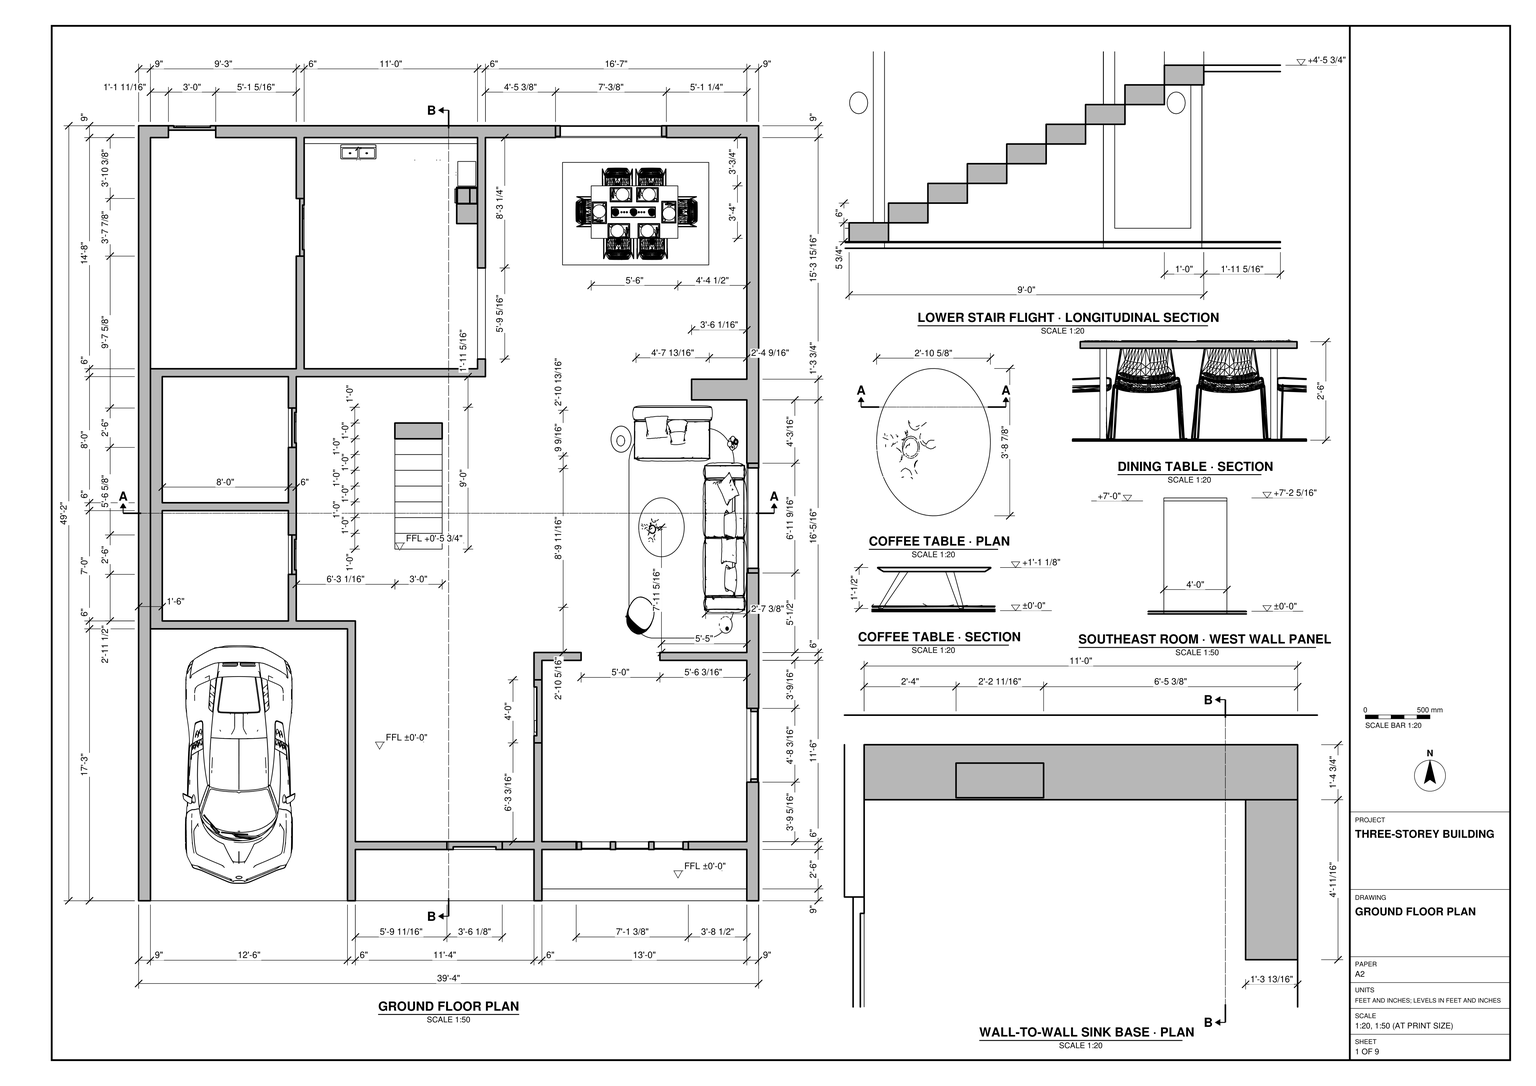
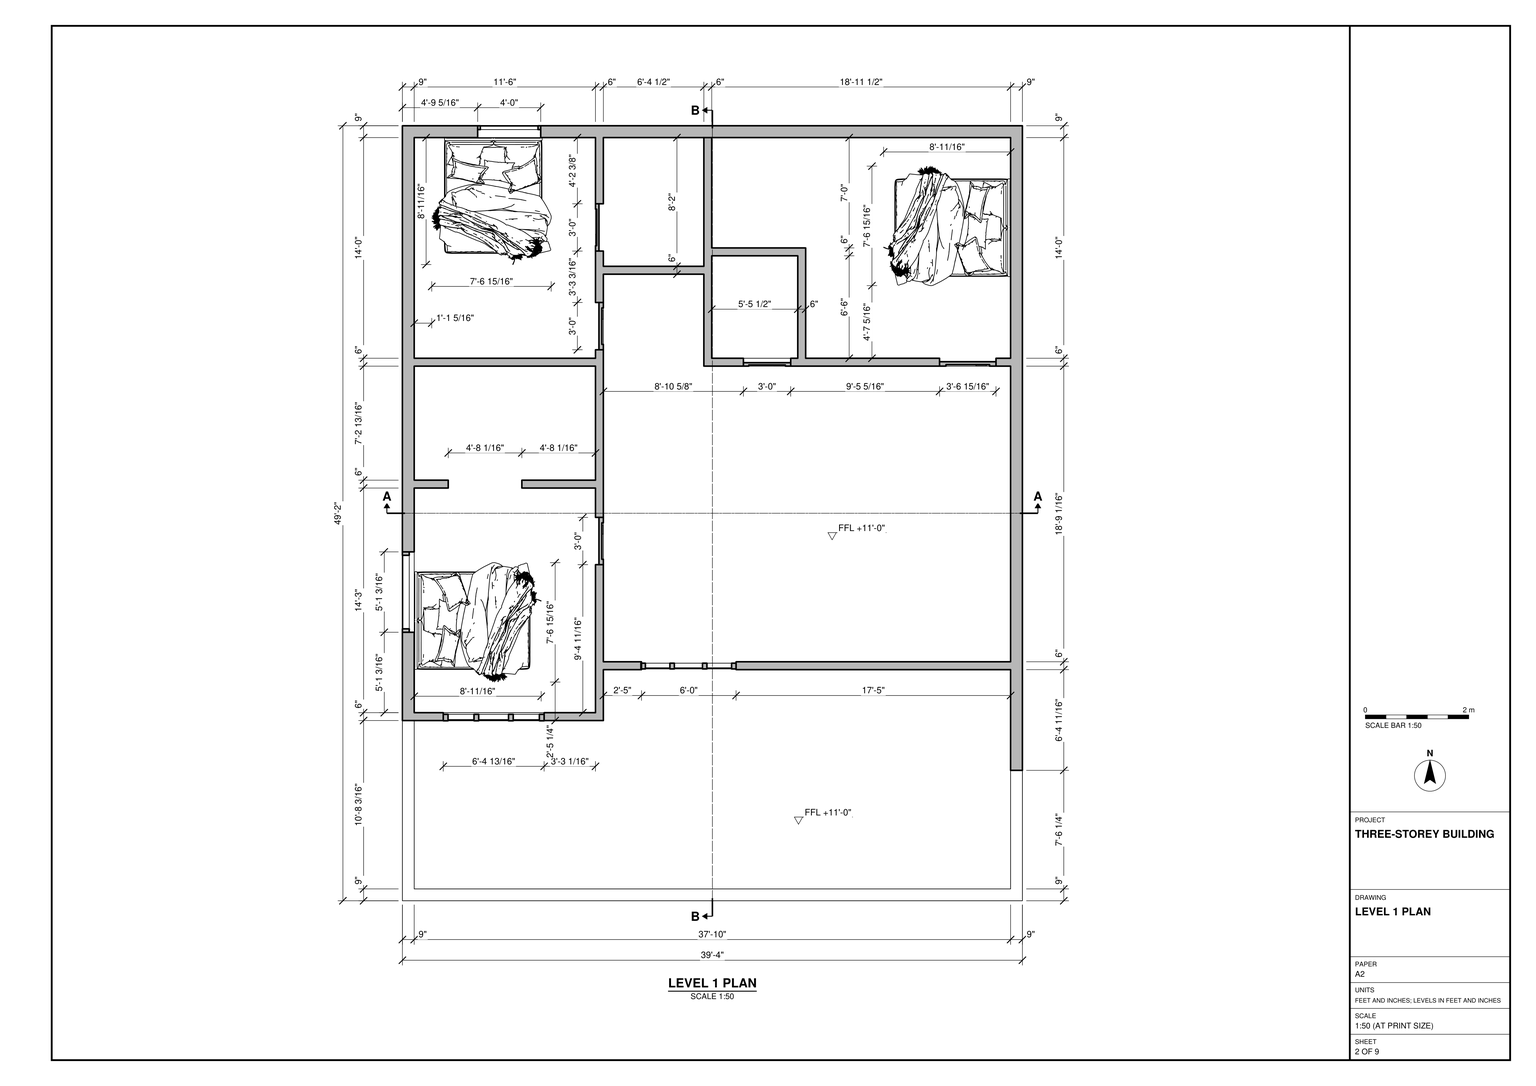
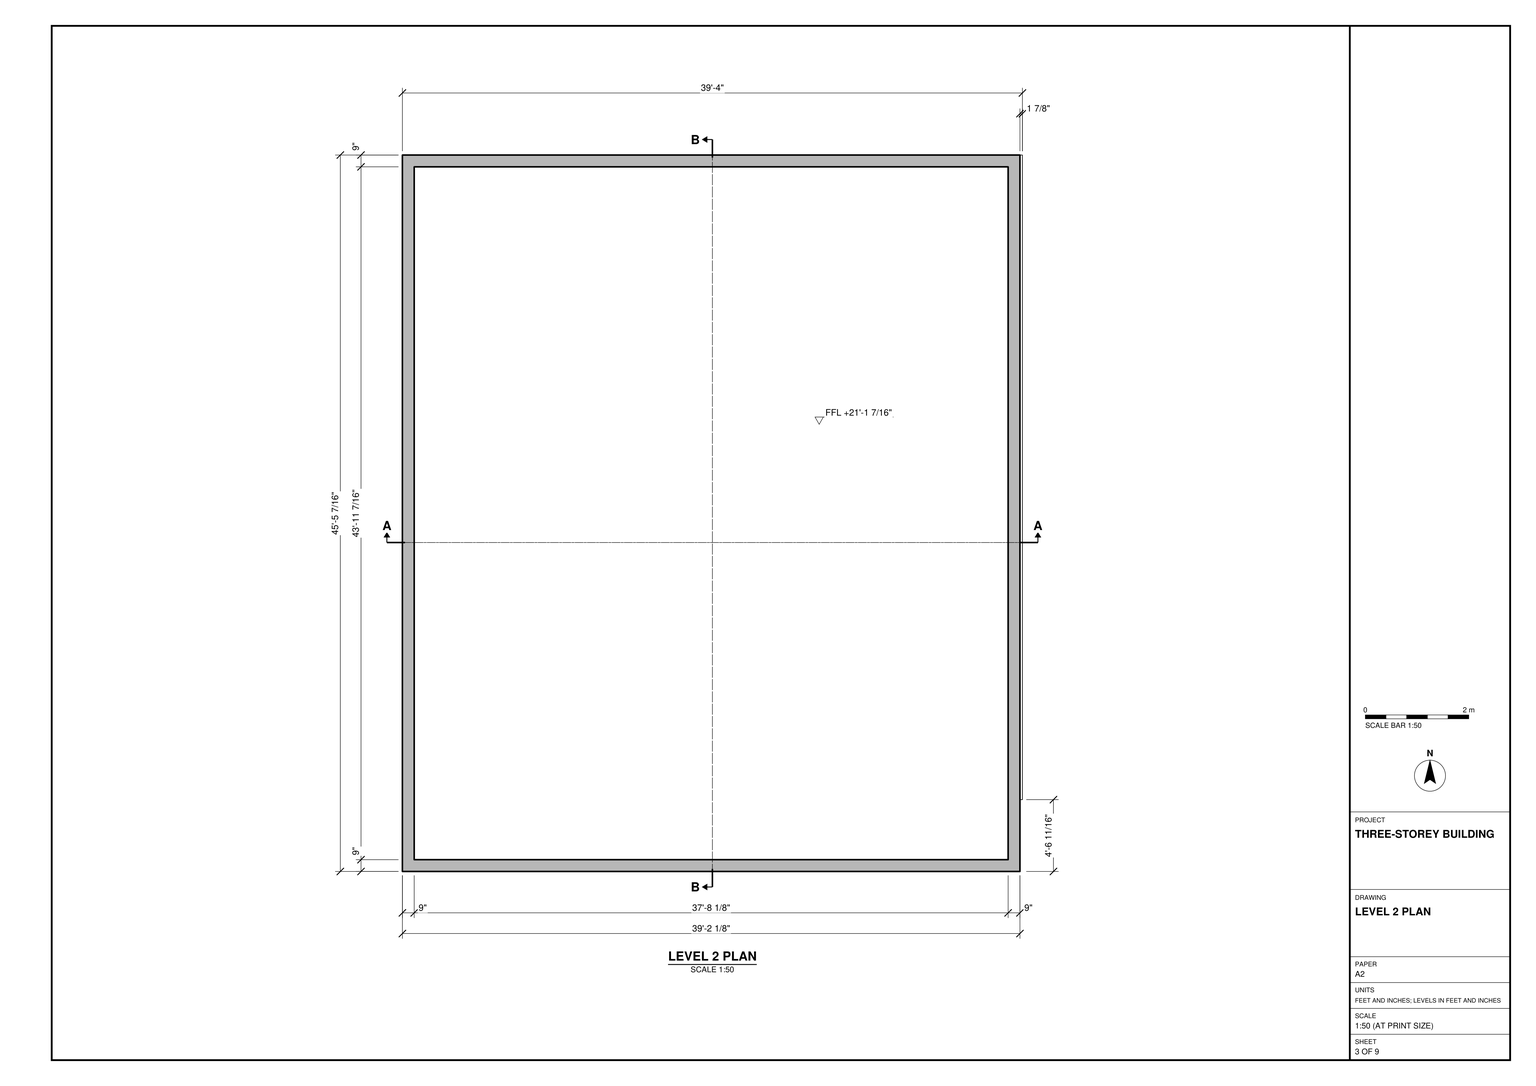
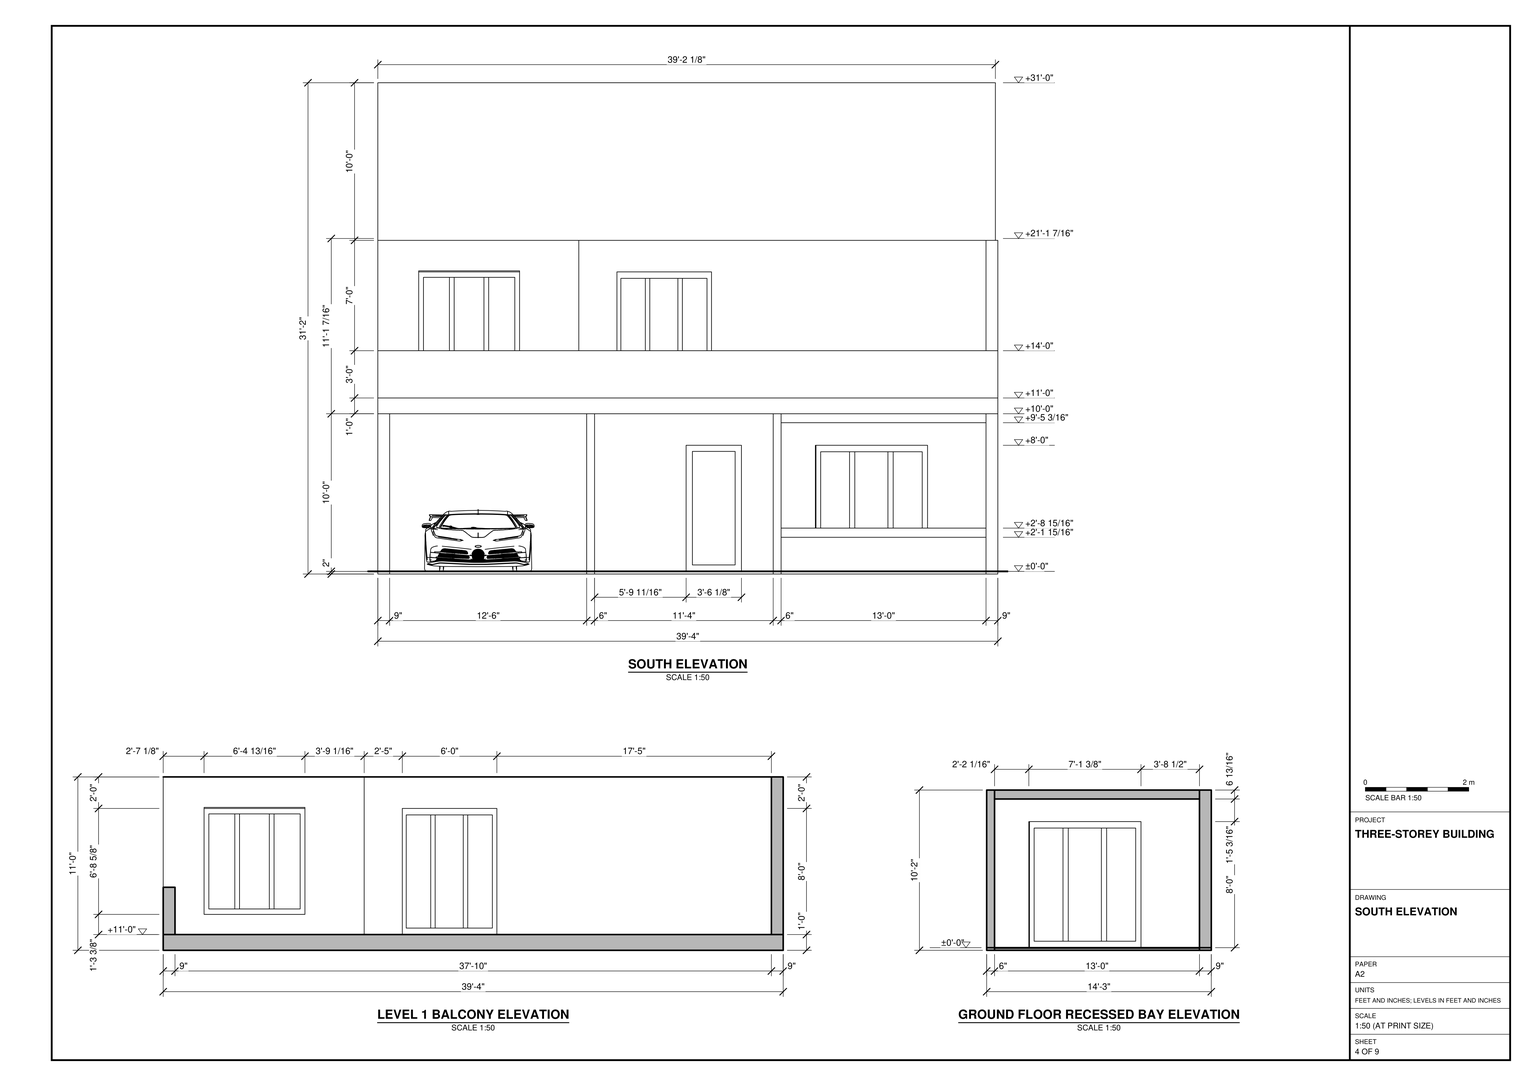
Build the three-storey residential building in SketchUp using task_files/diagram_01.pdf. Work in feet and inches. With north at the top of the plans, set out an overall east–west width of 39'-4" along X, a north–south depth of 49'-2" along Y and a total height of 31'-2". Use storey levels of ±0'-0", +10'-0" and +21'-1 7/16" relative to the ground floor.

Follow each floor plan for the wall positions and thicknesses, including the 9" perimeter walls and 6" partitions where indicated. Model the door and window openings, floor slabs, stairs, upper perimeter walls and roof edges as drawn. Preserve the stepped south edge of the enclosed rooms on the first upper floor rather than repeating the ground-floor layout.

On the ground floor, place the car in the southwest bay and the lower stair flight near the centre. Fit the kitchen with the wall-to-wall sink base and its return. Place the dining set in the northeast and arrange the sofas and coffee table farther south along the east side. Include the west wall panel in the southeast room. On the first upper floor, position and orient the beds to match the bedroom plan. Decor and loose items, including the car and appliances, may be any suitable library components.

Keep shell elements such as walls, slabs and roof separate as groups or components. Group each furniture or joinery piece separately and use components for repeated parts. Save one SketchUp model as output_files/three_storey_residential_building_and_its_furnishings.skp.

# SketchUp Ruby script. Lengths in inches.
U = 1.inch
M = Sketchup.active_model
def pt(a) = Geom::Point3d.new(a.map { |v| v * U })
def face(e, loops, mat)
  f = e.add_face(loops[0].map { |a| pt(a) })
  loops[1..].each { |l| e.add_face(l.map { |a| pt(a) }).erase! }
  f.material = f.back_material = mat if mat
  f
end
# faces: each face lists its corners as indices into pts; further lists are holes
def faces(e, pts, list, mat = nil) = list.each { |f| face(e, (f[0].is_a?(Array) ? f : [f]).map { |l| l.map { |i| pts[i] } }, mat) }
# xy, xz, yz: faces in a plane at the given z, y or x. An outline is a flat list of corners, or four numbers for a rectangle; further outlines are holes
def ring(l) = l.size == 4 ? [[l[0], l[1]], [l[2], l[1]], [l[2], l[3]], [l[0], l[3]]] : l.each_slice(2).to_a
def flat(e, list, mat, &to3) = list.each { |f| face(e, (f[0].is_a?(Array) ? f : [f]).map { |l| ring(l).map { |u, v| to3.(u, v) } }, mat) }
def xy(e, z, list, mat = nil) = flat(e, list, mat) { |x, y| [x, y, z] }
def xz(e, y, list, mat = nil) = flat(e, list, mat) { |x, z| [x, y, z] }
def yz(e, x, list, mat = nil) = flat(e, list, mat) { |y, z| [x, y, z] }
def lines(e, pts, list) = list.each { |a, b| e.add_line(pt(pts[a]), pt(pts[b])) }
# prism: a flat outline (further loops are holes) pulled along v
def prism(e, loops, v, mat = nil)
  f = face(e, loops, mat); d = Geom::Vector3d.new(v.map { |x| x * U })
  f.pushpull(f.normal.samedirection?(d) ? d.length : -d.length)
end
def box(e, o, s, mat = nil) = prism(e, [[o, [o[0] + s[0], o[1], o[2]], [o[0] + s[0], o[1] + s[1], o[2]], [o[0], o[1] + s[1], o[2]]]], [0, 0, s[2]], mat)
def at(x, y, z, deg = 0) = Geom::Transformation.translation(pt([x, y, z])) * Geom::Transformation.rotation(ORIGIN, Z_AXIS, deg.degrees)
def axes(o, x, y, z) = Geom::Transformation.new([*x, 0, *y, 0, *z, 0, *pt(o).to_a, 1])
def part(name) = M.definitions.add(name)
# library, detail: a bought-in or finely detailed component or shape, given as its bounding box
def library(name, o, s) = part(name).tap { |d| box(d.entities, o, s) }
def detail(e, o, s) = box(e.add_group.entities, o, s)
def put(e, d, t, mat = nil) = e.add_instance(d, t).tap { |i| i.material = mat if mat }
def group(e, t, mat = nil) = e.add_group.tap { |g| g.transformation = t; g.material = mat if mat }.entities
root = M.entities
M.materials.add("[Carrera Marble]").color = [207, 207, 207]
M.materials.add("[Color A01]").color = [255, 204, 204]
M.materials.add("[Color C08]").color = [102, 51, 0]
M.materials.add("[Color E01]").color = [255, 255, 204]
M.materials.add("[Color G01]").color = [204, 255, 204]
M.materials.add("[Color J01]").color = [229, 204, 255]
M.materials.add("[Color M08]").color = [30, 30, 30]
M.materials.add("[Concrete Pavers Block Multi]").color = [124, 140, 145]
M.materials.add("[Concrete Scored Jointless]").color = [140, 133, 127]
M.materials.add("[Formica Laminate Light]").color = [213, 189, 164]
M.materials.add("[Marble Carrara Gold Floor Tile]").color = [225, 223, 217]
M.materials.add("[Resin Blue]").color = [171, 210, 241]
M.materials.add("[Resin Turquoise]").color = [117, 218, 223]
M.materials.add("[Stone Coursed Rough]").color = [165, 160, 130]
M.materials.add("[Translucent Glass Blue]").color = [100, 149, 237]
M.materials.add("[Translucent Glass Gray]").color = [128, 128, 128]
M.materials.add("[Wood Floor]").color = [155, 105, 61]
c1 = library("L-shaped kitchen",[55.71,-118.11,21.3],[196.85,118.11,96.45])
c2 = library("28",[-28.6,-106.68,0],[90.94,96.67,40.97])
c3 = library("Sofa set Collection\#1",[635.72,692.31,0],[158.93,122.75,75.39])
c4 = library("skp3430",[-10.67,-22.6875,-0.04],[21.34,45.28,11.76])
c5 = library("Dining Set",[0,0,0],[111.37,78.0625,43.36])
c6 = part("Group\#7")
xy(c6.entities,0,[[0,0,36,6]])
xy(c6.entities,4.09,[[4.09,0,31.91,2.0625]],"[Color C08]")
xy(c6.entities,79.91,[[4.09,0,31.91,2.0625]],"[Color C08]")
xy(c6.entities,84,[[0,0,36,6]],"[Color C08]")
xz(c6.entities,0,[[[0,0,36,84],[4.09,4.09,31.91,79.91]]],"[Color C08]")
xz(c6.entities,0.25,[[26.54,38.97,27.4,39.08,28.2,39.41,28.88,39.9375,29.41,40.625,29.74,41.42,29.85,42.28,29.74,43.14,29.41,43.9375,28.88,44.625,28.2,45.15,27.4,45.48,26.54,45.59,25.68,45.48,24.89,45.15,24.2,44.625,23.67,43.9375,23.34,43.14,23.23,42.28,23.34,41.42,23.67,40.625,24.2,39.9375,24.89,39.41,25.68,39.08]],"[Color C08]")
xz(c6.entities,2.0625,[[[4.09,4.09,31.91,79.91],[26.54,38.97,25.68,39.08,24.89,39.41,24.2,39.9375,23.67,40.625,23.34,41.42,23.23,42.28,23.34,43.14,23.67,43.9375,24.2,44.625,24.89,45.15,25.68,45.48,26.54,45.59,27.4,45.48,28.2,45.15,28.88,44.625,29.41,43.9375,29.74,43.14,29.85,42.28,29.74,41.42,29.41,40.625,28.88,39.9375,28.2,39.41,27.4,39.08]]],"[Wood Floor]")
xz(c6.entities,6,[[0,0,36,84]])
yz(c6.entities,0,[[0,0,6,84]],"[Color C08]")
yz(c6.entities,4.09,[[0,4.09,2.0625,79.91]],"[Color C08]")
yz(c6.entities,31.91,[[0,4.09,2.0625,79.91]],"[Color C08]")
yz(c6.entities,36,[[0,0,6,84]],"[Color C08]")
p = [[25.68,2.0625,39.08],[26.54,2.0625,38.97],[26.54,0.25,38.97],[25.68,0.25,39.08],[27.4,2.0625,39.08],[27.4,0.25,39.08],
  [24.89,2.0625,39.41],[24.89,0.25,39.41],[28.2,2.0625,39.41],[28.2,0.25,39.41],[24.2,2.0625,39.9375],[24.2,0.25,39.9375],
  [28.88,2.0625,39.9375],[28.88,0.25,39.9375],[23.67,2.0625,40.625],[23.67,0.25,40.625],[29.41,2.0625,40.625],[29.41,0.25,40.625],
  [23.34,2.0625,41.42],[23.34,0.25,41.42],[29.74,2.0625,41.42],[29.74,0.25,41.42],[23.23,2.0625,42.28],[23.23,0.25,42.28],
  [29.85,2.0625,42.28],[29.85,0.25,42.28],[23.34,2.0625,43.14],[23.34,0.25,43.14],[29.74,2.0625,43.14],[29.74,0.25,43.14],
  [23.67,2.0625,43.9375],[23.67,0.25,43.9375],[29.41,2.0625,43.9375],[29.41,0.25,43.9375],[24.2,2.0625,44.625],[24.2,0.25,44.625],
  [28.88,2.0625,44.625],[28.88,0.25,44.625],[24.89,2.0625,45.15],[24.89,0.25,45.15],[28.2,2.0625,45.15],[28.2,0.25,45.15],
  [25.68,2.0625,45.48],[25.68,0.25,45.48],[27.4,2.0625,45.48],[27.4,0.25,45.48],[26.54,2.0625,45.59],[26.54,0.25,45.59]]
faces(c6.entities,p,[[0,1,2,3],[1,4,5,2],[6,0,3,7],[4,8,9,5],[10,6,7,11],[8,12,13,9],[14,10,11,15],[12,16,17,13],
  [18,14,15,19],[16,20,21,17],[22,18,19,23],[20,24,25,21],[26,22,23,27],[24,28,29,25],[30,26,27,31],[28,32,33,29],
  [34,30,31,35],[32,36,37,33],[38,34,35,39],[36,40,41,37],[42,38,39,43],[40,44,45,41],[46,42,43,47],[44,46,47,45]],"[Color C08]")
c7 = part("Group\#8")
box(c7.entities,[0,0,0],[36,12,6])
c8 = part("Group\#10")
put(c8.entities,c7,at(0,24,12))
put(c8.entities,c7,at(0,96,48))
put(c8.entities,c7,at(0,36,18))
put(c8.entities,c7,at(0,48,24))
put(c8.entities,c7,at(0,72,36))
put(c8.entities,c7,at(0,84,42))
put(c8.entities,c7,at(0,0,0))
put(c8.entities,c7,at(0,12,6))
put(c8.entities,c7,at(0,60,30))
c9 = part("Group\#14")
xy(c9.entities,0,[[0,0,8.11,83.5625]])
xy(c9.entities,3.3125,[[7.9,3.57,8.11,80]])
xy(c9.entities,3.3125,[[0,3.57,7.9,80]],"[Color C08]")
xy(c9.entities,44.6875,[[0,3.57,7.9,80],[7.9,3.57,8.11,80]])
xy(c9.entities,48,[[0,0,8.11,83.5625]],"[Color C08]")
xz(c9.entities,0,[[0,0,8.11,48]],"[Color C08]")
xz(c9.entities,3.57,[[7.9,3.3125,8.11,44.6875]])
xz(c9.entities,3.57,[[0,3.3125,7.9,44.6875]],"[Color C08]")
xz(c9.entities,80,[[7.9,3.3125,8.11,44.6875]])
xz(c9.entities,80,[[0,3.3125,7.9,44.6875]],"[Color C08]")
xz(c9.entities,83.5625,[[0,0,8.11,48]],"[Color C08]")
yz(c9.entities,0,[[[0,0,83.5625,48],[3.57,3.3125,80,44.6875]]],"[Color C08]")
yz(c9.entities,7.9,[[3.57,3.3125,80,44.6875]],"[Translucent Glass Gray]")
yz(c9.entities,8.11,[[[0,0,83.5625,48],[3.57,3.3125,80,44.6875]]],"[Color C08]")
c10 = library("Group\#11",[0,0,0],[343,572,6.8125])
c11 = part("Group\#12")
xy(c11.entities,0,[[0,0,77.625,5.875]])
xy(c11.entities,3.68,[[3.68,0,23.65,0.75],[23.65,0,27.29,5.875],[27.29,0,50.21,0.75],[50.21,0,53.85,5.875],[53.85,0,73.95,0.75],
  [3.68,0.75,23.65,5.875],[27.29,0.75,50.21,5.875],[53.85,0.75,73.95,5.875]],"[Color C08]")
xy(c11.entities,68.14,[[3.68,0,23.65,0.75],[23.65,0,27.29,5.875],[27.29,0,50.21,0.75],[50.21,0,53.85,5.875],[53.85,0,73.95,0.75],
  [3.68,0.75,23.65,5.875],[27.29,0.75,50.21,5.875],[53.85,0.75,73.95,5.875]])
xy(c11.entities,71.8125,[[0,0,77.625,5.875]],"[Color C08]")
xz(c11.entities,0,[[[0,0,77.625,71.8125],[3.68,3.68,73.95,68.14]],[23.65,3.68,27.29,68.14],[50.21,3.68,53.85,68.14]],"[Color C08]")
xz(c11.entities,0.75,[[3.68,3.68,23.65,68.14],[27.29,3.68,50.21,68.14],[53.85,3.68,73.95,68.14]],"[Translucent Glass Gray]")
xz(c11.entities,5.875,[[[0,0,77.625,71.8125],[3.68,3.68,73.95,68.14]],[23.65,3.68,27.29,68.14],[50.21,3.68,53.85,68.14]],"[Color C08]")
yz(c11.entities,0,[[0,0,5.875,71.8125]],"[Color C08]")
yz(c11.entities,3.68,[[0,3.68,0.75,68.14],[0.75,3.68,5.875,68.14]],"[Color C08]")
yz(c11.entities,23.65,[[0,3.68,0.75,68.14]])
yz(c11.entities,23.65,[[0.75,3.68,5.875,68.14]],"[Color C08]")
yz(c11.entities,27.29,[[0,3.68,0.75,68.14],[0.75,3.68,5.875,68.14]],"[Color C08]")
yz(c11.entities,50.21,[[0,3.68,0.75,68.14],[0.75,3.68,5.875,68.14]],"[Color C08]")
yz(c11.entities,53.85,[[0,3.68,0.75,68.14],[0.75,3.68,5.875,68.14]],"[Color C08]")
yz(c11.entities,73.95,[[0,3.68,0.75,68.14],[0.75,3.68,5.875,68.14]],"[Color C08]")
yz(c11.entities,77.625,[[0,0,5.875,71.8125]],"[Color C08]")
c12 = part("Group\#4")
xy(c12.entities,0,[[0,0,8.11,83.5625]])
xy(c12.entities,3.3125,[[7.9,3.57,8.11,80]])
xy(c12.entities,3.3125,[[0,3.57,7.9,80]],"[Color C08]")
xy(c12.entities,44.6875,[[0,3.57,7.9,80],[7.9,3.57,8.11,80]])
xy(c12.entities,48,[[0,0,8.11,83.5625]],"[Color C08]")
xz(c12.entities,0,[[0,0,8.11,48]],"[Color C08]")
xz(c12.entities,3.57,[[7.9,3.3125,8.11,44.6875]])
xz(c12.entities,3.57,[[0,3.3125,7.9,44.6875]],"[Color C08]")
xz(c12.entities,80,[[7.9,3.3125,8.11,44.6875]])
xz(c12.entities,80,[[0,3.3125,7.9,44.6875]],"[Color C08]")
xz(c12.entities,83.5625,[[0,0,8.11,48]],"[Color C08]")
yz(c12.entities,0,[[[0,0,83.5625,48],[3.57,3.3125,80,44.6875]]],"[Color C08]")
yz(c12.entities,7.9,[[3.57,3.3125,80,44.6875]],"[Translucent Glass Gray]")
yz(c12.entities,8.11,[[[0,0,83.5625,48],[3.57,3.3125,80,44.6875]]],"[Color C08]")
xy(root,252,[[0,44.5625,470.125,590]])
xy(root,253.4375,[[9,53.5625,461.125,581]])
xy(root,372,[[[0,44.5625,470.125,590],[9,53.5625,461.125,581]]])
xz(root,44.5625,[[0,252,470.125,372]],"[Color G01]")
xz(root,53.5625,[[9,253.4375,461.125,372]])
xz(root,581,[[9,253.4375,461.125,372]])
xz(root,590,[[0,252,470.125,372]])
yz(root,0,[[44.5625,252,590,372]],"[Color G01]")
yz(root,9,[[53.5625,253.4375,581,372]])
yz(root,461.125,[[53.5625,253.4375,581,372]])
yz(root,470.125,[[44.5625,252,590,372]],"[Color G01]")
# 1 loose lines left out
put(root,c1,axes([88.64,576.42,-21.03],[0.67056,0,0],[0,0.51559,0],[0,0,0.98757]))
put(root,c2,at(50.9375,591.01,132))
put(root,c3,axes([-237.95,1084.5,0],[0,-1.1131,0],[0.86,0,0],[0,0,1]))
put(root,c4,axes([76.36,103.91,0.17],[4,0,0],[0,4,0],[0,0,4]))
put(root,c5,at(322.6875,484.04,0))
put(root,c2,at(-1.01,195.0625,132,90))
put(root,c2,at(473.01,530.66,132,-90))
g1 = group(root,at(234.6875,39,0.24))
xy(g1,0,[[0,0,42.125,6]])
xy(g1,4.66,[[4.79,0,37.34,2.0625]],"[Color C08]")
xy(g1,91.1,[[4.79,0,37.34,2.0625]],"[Color C08]")
xy(g1,95.76,[[0,0,42.125,6]],"[Color C08]")
xz(g1,0,[[[0,0,42.125,95.76],[4.79,4.66,37.34,91.1]]],"[Color C08]")
xz(g1,2.0625,[[4.79,4.66,37.34,91.1]],"[Translucent Glass Blue]")
xz(g1,6,[[0,0,42.125,95.76]],"[Translucent Glass Blue]")
yz(g1,0,[[0,0,6,95.76]],"[Color C08]")
yz(g1,4.79,[[0,4.66,2.0625,91.1]],"[Color C08]")
yz(g1,37.34,[[0,4.66,2.0625,91.1]],"[Color C08]")
yz(g1,42.125,[[0,0,6,95.76]],"[Color C08]")
put(root,c6,axes([301,168.1875,0],[0,-1.33333,0],[1,0,0],[0,0,1.02728]))
put(root,c6,axes([126,490.74,0],[0,1.21875,0],[-0.56,0,0],[0,0,1]))
put(root,c6,axes([58.6875,590,0],[-1,0,0],[0,-0.56,0],[0,0,1]))
g2 = group(root,at(156.39,267.6875,-0.25))
box(g2,[0,108,52.0625],[74.6875,23.3125,1.9375])
put(g2,c8,at(38.6875,0,0))
put(g2,c8,at(36.4375,108,54,-180))
g3 = group(root,at(333.09,39,0))
xy(g3,0,[[0,0,85.39,5.875]])
xy(g3,4.92,[[4.05,0,26.02,0.75],[26.02,0,30.01,5.875],[30.01,0,55.24,0.75],[55.24,0,59.23,5.875],[59.23,0,81.34,0.75],
  [4.05,0.75,26.02,5.875],[30.01,0.75,55.24,5.875],[59.23,0.75,81.34,5.875]],"[Color C08]")
xy(g3,91.08,[[4.05,0,26.02,0.75],[26.02,0,30.01,5.875],[30.01,0,55.24,0.75],[55.24,0,59.23,5.875],[59.23,0,81.34,0.75],
  [4.05,0.75,26.02,5.875],[30.01,0.75,55.24,5.875],[59.23,0.75,81.34,5.875]])
xy(g3,96,[[0,0,85.39,5.875]],"[Color C08]")
xz(g3,0,[[[0,0,85.39,96],[4.05,4.92,81.34,91.08]],[26.02,4.92,30.01,91.08],[55.24,4.92,59.23,91.08]],"[Color C08]")
xz(g3,0.75,[[4.05,4.92,26.02,91.08],[30.01,4.92,55.24,91.08],[59.23,4.92,81.34,91.08]],"[Translucent Glass Gray]")
xz(g3,5.875,[[[0,0,85.39,96],[4.05,4.92,81.34,91.08]],[26.02,4.92,30.01,91.08],[55.24,4.92,59.23,91.08]],"[Color C08]")
yz(g3,0,[[0,0,5.875,96]],"[Color C08]")
yz(g3,4.05,[[0,4.92,0.75,91.08],[0.75,4.92,5.875,91.08]],"[Color C08]")
yz(g3,26.02,[[0,4.92,0.75,91.08]])
yz(g3,26.02,[[0.75,4.92,5.875,91.08]],"[Color C08]")
yz(g3,30.01,[[0,4.92,0.75,91.08],[0.75,4.92,5.875,91.08]],"[Color C08]")
yz(g3,55.24,[[0,4.92,0.75,91.08],[0.75,4.92,5.875,91.08]],"[Color C08]")
yz(g3,59.23,[[0,4.92,0.75,91.08],[0.75,4.92,5.875,91.08]],"[Color C08]")
yz(g3,81.34,[[0,4.92,0.75,91.08],[0.75,4.92,5.875,91.08]],"[Color C08]")
yz(g3,85.39,[[0,0,5.875,96]],"[Color C08]")
put(root,c9,axes([466.08,90.29,36],[0.6424,0,0],[0,0.6722,0],[0,0,1]))
put(root,c9,axes([401.74,581.89,36],[0,1,0],[-1.01,0,0],[0,0,1]))
put(root,c9,at(463.89,249.52,35.62))
put(root,c6,axes([120,248.47,0],[0,0.83333,0],[-0.56,0,0],[0,0,1]))
put(root,c6,axes([120,345.16,0],[0,0.83333,0],[-0.56,0,0],[0,0,1]))
put(root,c10,at(120,9.4375,113.1875))
put(root,c11,axes([31.12,136.99,147.35],[0.98929,0,0],[0,0.84,0],[0,0,1.12292]))
put(root,c9,axes([5.21,265.6,168],[-0.6424,0,0],[0,-0.73246,0],[0,0,1]))
put(root,c12,axes([105.31,587.08,168],[0,0.36,0],[-0.57442,0,0],[0,0,0.9864]))
put(root,c12,axes([200.85,588.1,201.9375],[0,0.234,0],[-0.28721,0,0],[0,0,0.51724]))
put(root,c6,axes([153,255.87,132],[0,1,0],[-0.56,0,0],[0,0,1]))
put(root,c6,axes([153,419.45,132],[0,1,0],[-0.56,0,0],[0,0,1]))
put(root,c6,axes([408.93,407,132],[1.19343,0,0],[0,0.56,0],[0,0,1]))
put(root,c6,axes([259.62,407,132],[1,0,0],[0,0.43999,0],[0,0,1]))
put(root,c6,axes([147,530.61,132],[0,-1,0],[0.43999,0,0],[0,0,1]))
put(root,c11,axes([181.58,176.48,132],[0.9333,0,0],[0,0.7476,0],[0,0,1.33681]))
g4 = group(root,at(0,0,-2),"[Color G01]")
xy(g4,0,[[0,0,0,590,9.3125,590,9.3125,581,9,581,9,0],[159,0,159,207,9.3125,207,9.3125,405,120,405,120,490.74,126,490.74,126,405,258,405,258,412.4,264,412.4,264,399,120,399,120,375.1,114,375.1,114,399,18,399,18,303,114,303,114,345.1,120,345.1,120,278.47,114,278.47,114,297,18,297,18,213,114,213,114,248.47,120,248.47,120,213,165,213,165,45,234.6875,45,234.6875,39,165,39,165,0],[301,0,301,39,276.8125,39,276.8125,45,301,45,301,120.1875,307,120.1875,307,45,333.57,45,333.57,39,307,39,307,0],[307,0,463,9],[463,0,463,39,418.48,39,418.48,45,463,45,463,90.29,472,90.29,472,0],
  [[307,9,307,39,333.57,39,333.57,45,307,45,307,120.1875,301,120.1875,301,45,165,45,165,213,120,213,120,399,264,399,264,581,317.34,581,317.34,590,401.89,590,401.89,581,463,581,463,397.04,420.9375,397.04,420.9375,381.29,463,381.29,463,189,396.83,189,396.83,183,463,183,463,146.46,472,146.46,472,90.29,463,90.29,463,45,418.48,45,418.48,39,463,39,463,9],[301,168.1875,307,168.1875,307,183,336.83,183,336.83,189,301,189]],[234.6875,39,276.8125,45],[463,146.46,463,183,396.83,183,396.83,189,463,189,463,333.08,472,333.08,472,146.46],[301,168.1875,301,189,336.83,189,336.83,183,307,183,307,168.1875],[114,248.47,120,278.47],
  [463,333.08,463,381.29,420.9375,381.29,420.9375,397.04,463,397.04,463,581,401.89,581,401.89,590,472,590,472,333.08],[114,345.1,120,375.1],[258,412.4,264,481.74],[258,481.74,258,581,126,581,126,534.62,120,534.62,120,581,58.6875,581,58.6875,590,317.34,590,317.34,581,264,581,264,481.74],[9.3125,581,22.6875,590]])
xy(g4,0,[[9,0,159,207]],"[Concrete Scored Jointless]")
xy(g4,0,[[165,0,301,39],[18,213,114,297],[18,303,114,399],[9.3125,405,9.3125,581,22.6875,581,22.6875,590,58.6875,590,58.6875,581,120,581,120,534.62,126,534.62,126,581,258,581,258,405,126,405,126,490.74,120,490.74,120,405]],"[Marble Carrara Gold Floor Tile]")
xy(g4,1.75,[[[307,9,463,9,463,39,418.48,39,418.48,45,463,45,463,90.29,472,90.29,472,146.46,463,146.46,463,183,396.83,183,396.83,189,463,189,463,381.29,420.9375,381.29,420.9375,397.04,463,397.04,463,581,401.89,581,401.89,590,317.34,590,317.34,581,264,581,264,399,120,399,120,213,165,213,165,45,301,45,301,120.1875,307,120.1875,307,45,333.57,45,333.57,39,307,39],[301,168.1875,301,189,336.83,189,336.83,183,307,183,307,168.1875]]])
xy(g4,2,[[0,0,9,0,9,581,9.3125,581,9.3125,590,0,590],[159,0,165,0,165,39,234.6875,39,234.6875,45,165,45,165,213,120,213,120,248.47,114,248.47,114,213,18,213,18,297,114,297,114,278.47,120,278.47,120,345.1,114,345.1,114,303,18,303,18,399,114,399,114,375.1,120,375.1,120,399,264,399,264,412.4,258,412.4,258,405,126,405,126,490.74,120,490.74,120,405,9.3125,405,9.3125,207,159,207],[301,0,307,0,307,39,333.57,39,333.57,45,307,45,307,120.1875,301,120.1875,301,45,276.8125,45,276.8125,39,301,39],[463,0,472,0,472,90.29,463,90.29,463,45,418.48,45,418.48,39,463,39],[234.6875,39,276.8125,45],
  [463,90.29,472,146.46],[463,146.46,472,146.46,472,333.08,463,333.08,463,189,396.83,189,396.83,183,463,183],[301,168.1875,307,168.1875,307,183,336.83,183,336.83,189,301,189],[9,207,9.3125,405],[114,248.47,120,278.47],
  [463,333.08,472,333.08,472,590,401.89,590,401.89,581,463,581,463,397.04,420.9375,397.04,420.9375,381.29,463,381.29],[114,345.1,120,375.1],[258,481.74,264,481.74,264,581,317.34,581,317.34,590,58.6875,590,58.6875,581,120,581,120,534.62,126,534.62,126,581,258,581],[9.3125,581,22.6875,590],[317.34,581,401.89,590]])
xy(g4,2,[[18,213,114,297],[18,303,114,399]],"[Carrera Marble]")
xy(g4,2,[[165,0,301,39]],"[Color G01]")
xy(g4,2,[[9,0,9.3125,207],[9.3125,0,159,207]],"[Concrete Scored Jointless]")
xy(g4,2,[[9.3125,405,120,405,120,490.74,126,490.74,126,405,258,405,258,581,126,581,126,534.62,120,534.62,120,581,58.6875,581,58.6875,590,22.6875,590,22.6875,581,9.3125,581],[258,412.4,264,481.74]],"[Formica Laminate Light]")
xy(g4,2,[[[307,9,463,9,463,39,418.48,39,418.48,45,463,45,463,183,396.83,183,396.83,189,463,189,463,381.29,420.9375,381.29,420.9375,397.04,463,397.04,463,581,264,581,264,399,120,399,120,213,165,213,165,45,301,45,301,120.1875,307,120.1875,307,45,333.57,45,333.57,39,307,39],[301,168.1875,301,189,336.83,189,336.83,183,307,183,307,168.1875]],[9,405,9.3125,581]],"[Marble Carrara Gold Floor Tile]")
xy(g4,27.9375,[[307,0,463,9]])
xy(g4,34.9375,[[307,0,463,9]],"[Color G01]")
xy(g4,38,[[463,90.29,472,146.46],[463,249.52,472,333.08],[317.34,581,401.89,590]])
xy(g4,86,[[463,90.29,472,146.46],[336.83,183,396.83,189],[114,248.47,120,278.47],[463,249.52,472,333.08],[114,345.1,120,375.1],
  [120,490.74,126,534.62],[22.6875,581,58.6875,590],[317.34,581,401.89,590]])
xy(g4,98,[[234.6875,39,276.8125,45],[333.57,39,418.48,45]])
xy(g4,122,[[9,0,159,207],[165,0,301,39],[307,0,463,39],[165,45,301,45,301,189,463,189,463,381.29,420.9375,381.29,420.9375,397.04,463,397.04,463,581,264,581,264,481.74,258,481.74,258,581,126,581,126,405,258,405,258,412.4,264,412.4,264,399,120,399,120,213,165,213],[18,213,114,297],
  [18,303,114,399],[9,405,120,581]])
xy(g4,122,[[[0,0,9,0,9,581,120,581,120,405,9,405,9,207,159,207,159,0,165,0,165,39,301,39,301,0,307,0,307,39,463,39,463,0,472,0,472,590,0,590],[165,45,165,213,120,213,120,399,264,399,264,412.4,258,412.4,258,405,126,405,126,581,258,581,258,481.74,264,481.74,264,581,463,581,463,397.04,420.9375,397.04,420.9375,381.29,463,381.29,463,189,301,189,301,45],[307,45,463,183],[18,303,114,399],[18,213,114,297]]],"[Color G01]")
xy(g4,134,[[0,0,0,137.1875,9,137.1875,9,9,463,9,463,99.27,472,99.27,472,0],[463,99.27,463,175.9375,254.03,175.9375,254.03,181.9375,463,181.9375,463,407,451.9,407,451.9,413,463,413,463,581,200.85,581,200.85,590,472,590,472,99.27],[0,137.1875,0,265.6,9,265.6,9,143.1875,107.91,143.1875,107.91,137.1875],[107.91,137.1875,107.91,143.1875,147,143.1875,147,255.87,153,255.87,153,181.9375,182.03,181.9375,182.03,175.9375,153,175.9375,153,137.1875],[0,265.6,0,590,105.31,590,105.31,581,9,581,9,413,147,413,147,419.45,153,419.45,153,291.87,147,291.87,147,314.1875,90.95,314.1875,90.95,320.1875,147,320.1875,147,407,9,407,9,320.1875,34.9,320.1875,34.9,314.1875,9,314.1875,9,265.6],
  [229.5,407,229.5,477,153,477,153,455.45,147,455.45,147,494.61,153,494.61,153,483,229.5,483,229.5,581,235.5,581,235.5,497,307,497,307,413,408.93,413,408.93,407,295.62,407,295.62,413,301,413,301,491,235.5,491,235.5,413,259.62,413,259.62,407],[235.5,413,301,491],[147,530.61,147,581,105.31,581,105.31,590,200.85,590,200.85,581,153,581,153,530.61]])
xy(g4,134,[[9,9,463,9,463,175.9375,254.03,175.9375,254.03,181.9375,463,181.9375,463,407,451.9,407,451.9,413,463,413,463,581,235.5,581,235.5,497,307,497,307,413,408.93,413,408.93,407,295.62,407,295.62,413,259.62,413,259.62,407,229.5,407,229.5,477,153,477,153,455.45,147,455.45,147,494.61,153,494.61,153,483,229.5,483,229.5,581,153,581,153,530.61,147,530.61,147,581,9,581,9,413,147,413,147,419.45,153,419.45,153,291.87,147,291.87,147,314.1875,90.95,314.1875,90.95,320.1875,147,320.1875,147,407,9,407,9,320.1875,34.9,320.1875,34.9,314.1875,9,314.1875,9,143.1875,147,143.1875,147,255.87,153,255.87,153,181.9375,182.03,181.9375,182.03,175.9375,153,175.9375,153,137.1875,9,137.1875]],"[Marble Carrara Gold Floor Tile]")
xy(g4,149.35,[[31.12,137.1875,107.91,143.1875]])
xy(g4,170,[[0,204.39,9,265.6],[57.31,581,105.31,590]])
xy(g4,170,[[0,0,472,0,472,99.27,463,99.27,463,9,9,9,9,137.1875,0,137.1875]],"[Color M08]")
xy(g4,203.9375,[[176.85,581,200.85,590]])
xy(g4,218,[[0,204.39,9,265.6],[147,255.87,153,291.87],[34.9,314.1875,90.95,320.1875],[259.62,407,295.62,413],[408.93,407,451.9,413],
  [147,419.45,153,455.45],[147,494.61,153,530.61],[57.31,581,105.31,590]])
xy(g4,228.76,[[176.85,581,200.85,590]])
xy(g4,230,[[182.03,175.9375,254.03,181.9375]])
xy(g4,230.8125,[[31.12,137.1875,107.91,143.1875]])
xy(g4,254,[[[463,99.27,472,99.27,472,590,0,590,0,137.1875,153,137.1875,153,175.9375,463,175.9375],[153,181.9375,153,477,229.5,477,229.5,407,463,407,463,181.9375],[307,413,307,497,235.5,497,235.5,581,229.5,581,229.5,483,153,483,153,581,463,581,463,413],[9,143.1875,147,314.1875],[9,413,147,581],[9,320.1875,147,407],[235.5,413,301,491]]],"[Color E01]")
xz(g4,0,[[0,0,9,2],[301,0,307,2]])
xz(g4,0,[[9,0,159,2],[159,0,165,2],[165,0,301,2],[307,0,463,2],[463,0,472,2],
  [0,2,9,122],[159,2,165,122],[301,2,307,122],[463,2,472,122],[307,27.9375,463,34.9375],
  [0,122,472,134]],"[Color G01]")
xz(g4,0,[[307,2,463,27.9375]],"[Stone Coursed Rough]")
xz(g4,0,[[0,134,472,170]],"[Translucent Glass Blue]")
xz(g4,9,[[307,0,463,1.75],[307,1.75,463,2],[307,2,463,27.9375],[307,27.9375,463,34.9375]])
xz(g4,9,[[9,134,463,170]],"[Translucent Glass Blue]")
xz(g4,39,[[307,0,333.57,1.75],[418.48,0,463,1.75],[307,1.75,333.57,2],[418.48,1.75,463,2]])
xz(g4,39,[[165,2,234.6875,2,234.6875,98,276.8125,98,276.8125,2,301,2,301,122,165,122],[307,2,333.57,2,333.57,98,418.48,98,418.48,2,463,2,463,122,307,122]],"[Color G01]")
xz(g4,39,[[165,0,234.6875,2],[234.6875,0,276.8125,2],[276.8125,0,301,2]],"[Marble Carrara Gold Floor Tile]")
xz(g4,45,[[165,0,185.25,1.75],[185.25,0,234.6875,1.75],[234.6875,0,271.8125,1.75],[271.8125,0,276.8125,1.75],[276.8125,0,301,1.75],
  [307,0,333.57,1.75],[418.48,0,463,1.75],[165,1.75,185.25,2],[185.25,1.75,234.6875,2],[234.6875,1.75,271.8125,2],
  [271.8125,1.75,276.8125,2],[276.8125,1.75,301,2],[307,1.75,333.57,2],[418.48,1.75,463,2],[165,2,165,122,301,122,301,2,276.8125,2,276.8125,98,234.6875,98,234.6875,2]])
xz(g4,45,[[307,2,307,122,463,122,463,2,418.48,2,418.48,98,333.57,98,333.57,2]],"[Color J01]")
xz(g4,90.29,[[463,0,472,1.75],[463,1.75,472,2],[463,38,472,86]])
xz(g4,99.27,[[463,134,472,170]])
xz(g4,99.27,[[463,170,472,254]],"[Color G01]")
xz(g4,120.1875,[[301,0,307,1.75],[301,1.75,307,2],[301,2,301,88.29,307,86,307,2]])
xz(g4,137.1875,[[0,134,9,170]])
xz(g4,137.1875,[[[9,134,153,134,153,254,0,254,0,170,9,170],[31.12,149.35,107.91,230.8125]]],"[Color G01]")
xz(g4,143.1875,[[[9,134,147,254],[31.12,149.35,107.91,230.8125]]],"[Resin Turquoise]")
xz(g4,146.46,[[463,0,472,1.75],[463,1.75,472,2],[463,38,472,86]])
xz(g4,168.1875,[[301,0,307,1.75],[301,1.75,307,2],[301,2,301,88.29,307,86,307,2]])
xz(g4,175.9375,[[153,134,182.03,134,182.03,230,254.03,230,254.03,134,463,134,463,254,153,254]],"[Color G01]")
xz(g4,181.9375,[[153,134,153,254,463,254,463,134,254.03,134,254.03,230,182.03,230,182.03,134]],"[Color E01]")
xz(g4,183,[[307,0,336.83,1.75],[396.83,0,463,1.75],[307,1.75,336.83,2],[396.83,1.75,463,2]])
xz(g4,183,[[307,2,336.83,2,336.83,86,396.83,86,396.83,2,463,2,463,122,307,122]],"[Color J01]")
xz(g4,189,[[301,0,336.83,1.75],[396.83,0,463,1.75],[301,1.75,336.83,2],[396.83,1.75,463,2]])
xz(g4,189,[[301,2,301,122,463,122,463,2,396.83,2,396.83,86,336.83,86,336.83,2]],"[Resin Blue]")
xz(g4,204.39,[[0,170,9,218]])
xz(g4,207,[[9.3125,0,159,2]])
xz(g4,207,[[9,2,159,122]],"[Color G01]")
xz(g4,207,[[9,0,9.3125,2]],"[Concrete Scored Jointless]")
xz(g4,213,[[120,0,165,1.75],[120,1.75,165,2],[120,2,165,122]])
xz(g4,213,[[18,2,114,122]],"[Color A01]")
xz(g4,213,[[18,0,114,2]],"[Marble Carrara Gold Floor Tile]")
xz(g4,248.47,[[114,0,120,2],[114,2,120,86]])
xz(g4,249.52,[[463,38,472,86]])
xz(g4,255.87,[[147,134,153,218]])
xz(g4,265.6,[[0,170,9,218]])
xz(g4,278.47,[[114,0,120,2],[114,2,120,86]])
xz(g4,291.87,[[147,134,153,218]])
xz(g4,297,[[18,2,114,122]],"[Color A01]")
xz(g4,297,[[18,0,114,2]],"[Marble Carrara Gold Floor Tile]")
xz(g4,303,[[18,2,114,122]],"[Concrete Pavers Block Multi]")
xz(g4,303,[[18,0,114,2]],"[Marble Carrara Gold Floor Tile]")
xz(g4,314.1875,[[9,134,34.9,134,34.9,218,90.95,218,90.95,134,147,134,147,254,9,254]],"[Resin Turquoise]")
xz(g4,320.1875,[[9,134,9,254,147,254,147,134,90.95,134,90.95,218,34.9,218,34.9,134]])
xz(g4,333.08,[[463,0,472,2],[463,38,472,86]])
xz(g4,345.1,[[114,0,120,2],[114,2,120,86]])
xz(g4,375.1,[[114,0,120,2],[114,2,120,86]])
xz(g4,381.29,[[420.9375,0,463,1.75],[420.9375,1.75,463,2]])
xz(g4,381.29,[[420.9375,2,463,122]],"[Resin Blue]")
xz(g4,397.04,[[420.9375,0,463,1.75],[420.9375,1.75,463,2]])
xz(g4,397.04,[[420.9375,2,463,122]],"[Resin Turquoise]")
xz(g4,399,[[120,0,264,1.75],[120,1.75,264,2]])
xz(g4,399,[[18,2,114,122]],"[Concrete Pavers Block Multi]")
xz(g4,399,[[18,0,114,2]],"[Marble Carrara Gold Floor Tile]")
xz(g4,399,[[120,2,264,122]],"[Resin Blue]")
xz(g4,405,[[126,2,258,122]],"[Color A01]")
xz(g4,405,[[9,2,120,122]],"[Color J01]")
xz(g4,405,[[9.3125,0,120,2],[126,0,258,2]],"[Marble Carrara Gold Floor Tile]")
xz(g4,407,[[9,134,147,254],[229.5,134,259.62,134,259.62,218,295.62,218,295.62,134,408.93,134,408.93,218,451.9,218,451.9,134,463,134,463,254,229.5,254]],"[Color E01]")
xz(g4,412.4,[[258,0,264,2]])
xz(g4,412.4,[[258,2,264,122]],"[Resin Turquoise]")
xz(g4,413,[[9,134,147,254]],"[Color E01]")
xz(g4,413,[[235.5,134,235.5,254,301,254,301,134,295.62,134,295.62,218,259.62,218,259.62,134]],"[Concrete Pavers Block Multi]")
xz(g4,413,[[307,134,307,254,463,254,463,134,451.9,134,451.9,218,408.93,218,408.93,134]],"[Resin Turquoise]")
xz(g4,419.45,[[147,134,153,218]])
xz(g4,455.45,[[147,134,153,218]])
xz(g4,477,[[153,134,229.5,254]],"[Color E01]")
xz(g4,481.74,[[258,0,264,2]])
xz(g4,481.74,[[258,2,264,122]],"[Resin Turquoise]")
xz(g4,483,[[153,134,229.5,254]],"[Concrete Pavers Block Multi]")
xz(g4,490.74,[[120,2,126,86]])
xz(g4,490.74,[[120,0,126,2]],"[Marble Carrara Gold Floor Tile]")
xz(g4,491,[[235.5,134,301,254]],"[Concrete Pavers Block Multi]")
xz(g4,494.61,[[147,134,153,218]])
xz(g4,497,[[235.5,134,307,254]],"[Resin Turquoise]")
xz(g4,530.61,[[147,134,153,218]])
xz(g4,534.62,[[120,2,126,30.25],[120,30.25,126,86]])
xz(g4,534.62,[[120,0,126,2]],"[Marble Carrara Gold Floor Tile]")
xz(g4,581,[[9,0,9.3125,2],[264,0,317.34,1.75],[401.89,0,463,1.75],[264,1.75,317.34,2],[401.89,1.75,463,2],
  [126,2,258,30.25],[229.5,134,235.5,254]])
xz(g4,581,[[126,30.25,258,122]],"[Color A01]")
xz(g4,581,[[[9,134,147,254],[57.31,170,105.31,218]]],"[Color E01]")
xz(g4,581,[[9,2,22.6875,2,22.6875,86,58.6875,86,58.6875,2,120,2,120,122,9,122]],"[Color J01]")
xz(g4,581,[[[153,134,229.5,254],[176.85,203.9375,200.85,228.76]]],"[Concrete Pavers Block Multi]")
xz(g4,581,[[9.3125,0,22.6875,2],[58.6875,0,120,2],[126,0,258,2]],"[Marble Carrara Gold Floor Tile]")
xz(g4,581,[[[264,2,463,122],[317.34,38,401.89,86]],[235.5,134,463,254]],"[Resin Turquoise]")
xz(g4,590,[[317.34,0,401.89,1.75],[401.89,0,472,2],[317.34,1.75,401.89,2]])
xz(g4,590,[[0,0,9.3125,2],[9.3125,0,22.6875,2],[22.6875,0,58.6875,2],[58.6875,0,317.34,2],[[0,2,0,122,472,122,472,2,58.6875,2,58.6875,86,22.6875,86,22.6875,2],[317.34,38,401.89,86]],
  [0,122,472,134],[[0,134,472,254],[57.31,170,105.31,218],[176.85,203.9375,200.85,228.76]]],"[Color G01]")
yz(g4,0,[[0,0,590,2],[0,2,590,122],[0,122,590,134],[[137.1875,134,590,254],[204.39,170,265.6,218]]],"[Color G01]")
yz(g4,0,[[0,134,137.1875,170]],"[Translucent Glass Blue]")
yz(g4,9,[[207,0,405,2],[405,0,581,2],[207,2,405,122]])
yz(g4,9,[[320.1875,134,407,254],[413,134,581,254]],"[Color E01]")
yz(g4,9,[[0,2,207,122]],"[Color G01]")
yz(g4,9,[[405,2,581,122]],"[Color J01]")
yz(g4,9,[[0,0,207,2]],"[Concrete Scored Jointless]")
yz(g4,9,[[[143.1875,134,314.1875,254],[204.39,170,265.6,218]]],"[Resin Turquoise]")
yz(g4,9,[[9,134,137.1875,170]],"[Translucent Glass Blue]")
yz(g4,9.3125,[[207,0,405,2],[581,0,590,2]])
yz(g4,9.3125,[[405,0,581,2]],"[Marble Carrara Gold Floor Tile]")
yz(g4,18,[[213,2,297,122]],"[Color A01]")
yz(g4,18,[[303,2,399,122]],"[Concrete Pavers Block Multi]")
yz(g4,18,[[213,0,297,2],[303,0,399,2]],"[Marble Carrara Gold Floor Tile]")
yz(g4,22.6875,[[581,2,590,86]])
yz(g4,22.6875,[[581,0,590,2]],"[Marble Carrara Gold Floor Tile]")
yz(g4,31.12,[[137.1875,149.35,143.1875,230.8125]])
yz(g4,34.9,[[314.1875,134,320.1875,218]])
yz(g4,57.31,[[581,170,590,218]])
yz(g4,58.6875,[[581,2,590,30.25],[581,30.25,590,86]])
yz(g4,58.6875,[[581,0,590,2]],"[Marble Carrara Gold Floor Tile]")
yz(g4,90.95,[[314.1875,134,320.1875,218]])
yz(g4,105.31,[[581,170,590,218]])
yz(g4,107.91,[[137.1875,149.35,143.1875,230.8125]])
yz(g4,114,[[213,2,213,122,297,122,297,2,278.47,2,278.47,86,248.47,86,248.47,2]],"[Color A01]")
yz(g4,114,[[303,2,303,122,399,122,399,2,375.1,2,375.1,86,345.1,86,345.1,2]],"[Concrete Pavers Block Multi]")
yz(g4,114,[[213,0,248.47,2],[248.47,0,278.47,2],[278.47,0,297,2],[303,0,345.1,2],[345.1,0,375.1,2],
  [375.1,0,399,2]],"[Marble Carrara Gold Floor Tile]")
yz(g4,120,[[213,0,248.47,1.75],[248.47,0,278.47,1.75],[278.47,0,345.1,1.75],[345.1,0,375.1,1.75],[375.1,0,399,1.75],
  [213,1.75,248.47,2],[248.47,1.75,278.47,2],[278.47,1.75,345.1,2],[345.1,1.75,375.1,2],[375.1,1.75,399,2]])
yz(g4,120,[[405,2,405,122,581,122,581,2,534.62,2,534.62,86,490.74,86,490.74,2]],"[Color J01]")
yz(g4,120,[[405,0,490.74,2],[534.62,0,581,2]],"[Marble Carrara Gold Floor Tile]")
yz(g4,120,[[213,2,248.47,2,248.47,86,278.47,86,278.47,2,345.1,2,345.1,86,375.1,86,375.1,2,399,2,399,122,213,122]],"[Resin Blue]")
yz(g4,126,[[534.62,2,581,30.25]])
yz(g4,126,[[405,2,490.74,2,490.74,86,534.62,86,534.62,30.25,581,30.25,581,122,405,122]],"[Color A01]")
yz(g4,126,[[405,0,490.74,2],[534.62,0,581,2]],"[Marble Carrara Gold Floor Tile]")
yz(g4,147,[[320.1875,134,407,254],[413,134,413,254,581,254,581,134,530.61,134,530.61,218,494.61,218,494.61,134,455.45,134,455.45,218,419.45,218,419.45,134]],"[Color E01]")
yz(g4,147,[[143.1875,134,143.1875,254,314.1875,254,314.1875,134,291.87,134,291.87,218,255.87,218,255.87,134]],"[Resin Turquoise]")
yz(g4,153,[[137.1875,134,175.9375,254],[483,134,494.61,254]])
yz(g4,153,[[181.9375,134,255.87,134,255.87,218,291.87,218,291.87,134,419.45,134,419.45,218,455.45,218,455.45,134,477,134,477,254,181.9375,254]],"[Color E01]")
yz(g4,153,[[530.61,134,581,134,581,254,494.61,254,494.61,218,530.61,218]],"[Concrete Pavers Block Multi]")
yz(g4,159,[[0,2,207,122]],"[Color G01]")
yz(g4,159,[[0,0,207,2]],"[Concrete Scored Jointless]")
yz(g4,165,[[45,0,213,1.75],[45,1.75,213,2]])
yz(g4,165,[[0,2,39,122]],"[Color G01]")
yz(g4,165,[[0,0,39,2]],"[Marble Carrara Gold Floor Tile]")
yz(g4,165,[[45,2,213,122]],"[Resin Blue]")
yz(g4,176.85,[[581,203.9375,590,206],[581,206,590,228.76]])
yz(g4,182.03,[[175.9375,134,181.9375,139.68],[175.9375,139.68,181.9375,230]])
yz(g4,200.85,[[581,203.9375,590,228.76]])
yz(g4,229.5,[[407,134,477,254]],"[Color E01]")
yz(g4,229.5,[[483,134,581,254]],"[Concrete Pavers Block Multi]")
yz(g4,234.6875,[[39,0,45,2],[39,2,45,98]])
yz(g4,235.5,[[413,134,491,254]],"[Concrete Pavers Block Multi]")
yz(g4,235.5,[[497,134,581,254]],"[Resin Turquoise]")
yz(g4,254.03,[[175.9375,134,181.9375,230]])
yz(g4,258,[[405,2,412.4,122]])
yz(g4,258,[[481.74,2,581,122]],"[Color A01]")
yz(g4,258,[[405,0,412.4,2],[412.4,0,481.74,2],[481.74,0,581,2]],"[Marble Carrara Gold Floor Tile]")
yz(g4,259.62,[[407,134,413,218]])
yz(g4,264,[[399,0,412.4,1.75],[412.4,0,481.74,1.75],[481.74,0,581,1.75],[399,1.75,412.4,2],[412.4,1.75,481.74,2],
  [481.74,1.75,581,2]])
yz(g4,264,[[399,2,412.4,122],[481.74,2,581,122]],"[Resin Turquoise]")
yz(g4,276.8125,[[39,0,45,2],[39,2,45,98]])
yz(g4,295.62,[[407,134,413,218]])
yz(g4,301,[[45,0,120.1875,1.75],[168.1875,0,189,1.75],[45,1.75,120.1875,2],[168.1875,1.75,189,2]])
yz(g4,301,[[0,2,39,122]],"[Color G01]")
yz(g4,301,[[413,134,491,254]],"[Concrete Pavers Block Multi]")
yz(g4,301,[[0,0,39,2]],"[Marble Carrara Gold Floor Tile]")
yz(g4,301,[[45,2,45,122,189,122,189,2,168.1875,2,168.1875,88.29,120.1875,88.29,120.1875,2]],"[Resin Blue]")
yz(g4,307,[[0,0,9,2],[9,0,39,1.75],[45,0,120.1875,1.75],[168.1875,0,183,1.75],[9,1.75,39,2],
  [45,1.75,120.1875,2],[168.1875,1.75,183,2],[0,2,9,27.9375],[0,27.9375,9,34.9375]])
yz(g4,307,[[9,2,39,2,39,122,0,122,0,34.9375,9,34.9375]],"[Color G01]")
yz(g4,307,[[45,2,120.1875,2,120.1875,86,168.1875,86,168.1875,2,183,2,183,122,45,122]],"[Color J01]")
yz(g4,307,[[413,134,497,254]],"[Resin Turquoise]")
yz(g4,317.34,[[581,0,590,1.75],[581,1.75,590,2],[581,38,590,86]])
yz(g4,333.57,[[39,0,45,1.75],[39,1.75,45,2],[39,2,45,98]])
yz(g4,336.83,[[183,0,189,1.75],[183,1.75,189,2],[183,2,189,86]])
yz(g4,396.83,[[183,0,189,1.75],[183,1.75,189,2],[183,2,189,86]])
yz(g4,401.89,[[581,0,590,1.75],[581,1.75,590,2],[581,38,590,86]])
yz(g4,408.93,[[407,134,413,218]])
yz(g4,418.48,[[39,0,45,1.75],[39,1.75,45,2],[39,2,45,98]])
yz(g4,420.9375,[[381.29,0,397.04,1.75],[381.29,1.75,397.04,2]])
yz(g4,420.9375,[[381.29,2,397.04,122]],"[Resin Blue]")
yz(g4,451.9,[[407,134,413,218]])
yz(g4,463,[[0,0,9,2],[9,0,39,1.75],[45,0,90.29,1.75],[146.46,0,183,1.75],[189,0,333.08,1.75],
  [333.08,0,381.29,1.75],[397.04,0,581,1.75],[9,1.75,39,2],[45,1.75,90.29,2],[146.46,1.75,183,2],
  [189,1.75,333.08,2],[333.08,1.75,381.29,2],[397.04,1.75,581,2],[0,2,9,27.9375],[0,27.9375,9,34.9375],
  [99.27,134,175.9375,254]])
yz(g4,463,[[181.9375,134,407,254]],"[Color E01]")
yz(g4,463,[[9,2,9,34.9375,0,34.9375,0,122,39,122,39,2]],"[Color G01]")
yz(g4,463,[[[45,2,183,122],[90.29,38,146.46,86]]],"[Color J01]")
yz(g4,463,[[[189,2,381.29,122],[249.52,38,333.08,86]]],"[Resin Blue]")
yz(g4,463,[[397.04,2,581,122],[413,134,581,254]],"[Resin Turquoise]")
yz(g4,463,[[9,134,99.27,170]],"[Translucent Glass Blue]")
yz(g4,472,[[0,0,90.29,2],[90.29,0,146.46,1.75],[146.46,0,333.08,2],[333.08,0,590,2],[90.29,1.75,146.46,2]])
yz(g4,472,[[[0,2,590,122],[249.52,38,333.08,86],[90.29,38,146.46,86]],[0,122,590,134],[99.27,134,590,254]],"[Color G01]")
yz(g4,472,[[0,134,99.27,170]],"[Translucent Glass Blue]")
# 1 loose lines left out
p = [[301,120.1875,88.29],[301,168.1875,88.29],[307,168.1875,86],[307,120.1875,86],[307,168.3125,86],[301,168.3125,88.29]]
faces(g4,p,[[0,1,2,3],[4,2,1,5]])
